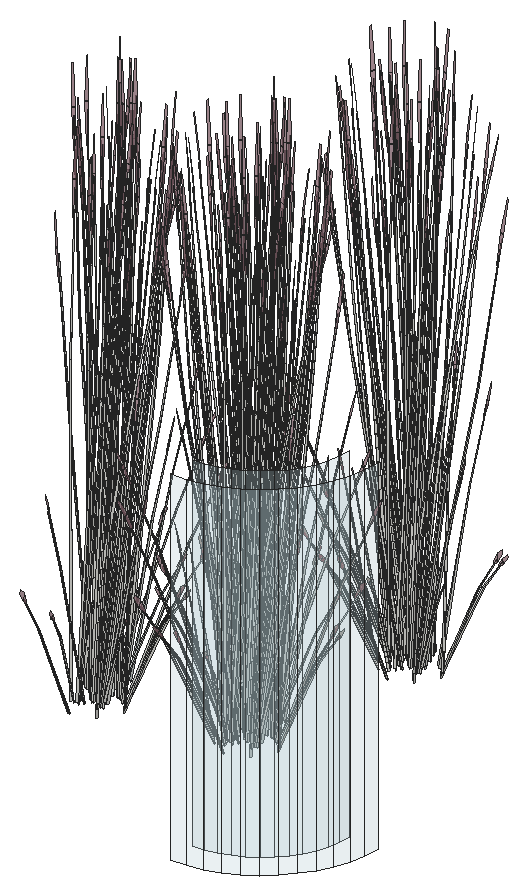
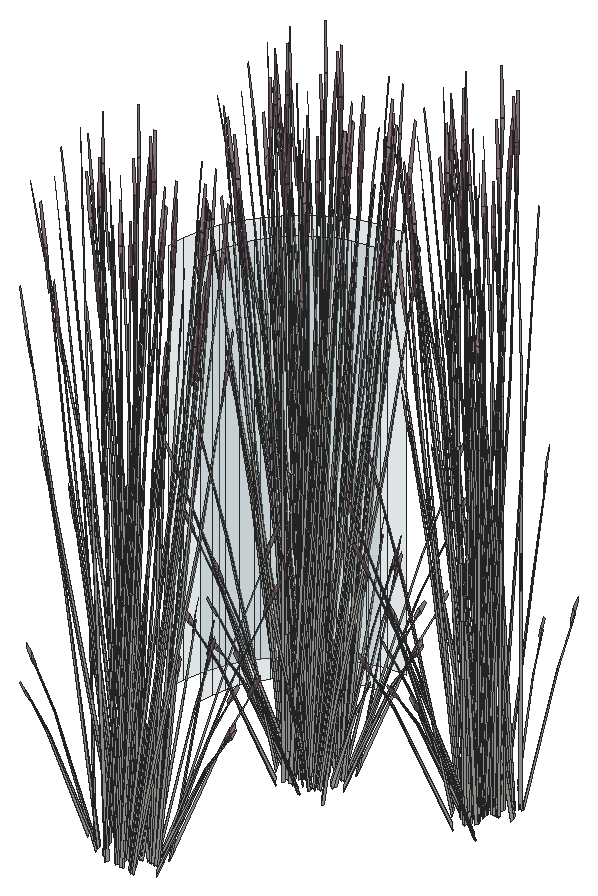
# SketchUp Ruby script. Lengths in inches.
U = 1.inch
M = Sketchup.active_model
def pt(a) = Geom::Point3d.new(a.map { |v| v * U })
def face(e, loops, mat)
  f = e.add_face(loops[0].map { |a| pt(a) })
  loops[1..].each { |l| e.add_face(l.map { |a| pt(a) }).erase! }
  f.material = f.back_material = mat if mat
  f
end
# faces: each face lists its corners as indices into pts; further lists are holes
def faces(e, pts, list, mat = nil) = list.each { |f| face(e, (f[0].is_a?(Array) ? f : [f]).map { |l| l.map { |i| pts[i] } }, mat) }
# xy, xz, yz: faces in a plane at the given z, y or x. An outline is a flat list of corners, or four numbers for a rectangle; further outlines are holes
def ring(l) = l.size == 4 ? [[l[0], l[1]], [l[2], l[1]], [l[2], l[3]], [l[0], l[3]]] : l.each_slice(2).to_a
def flat(e, list, mat, &to3) = list.each { |f| face(e, (f[0].is_a?(Array) ? f : [f]).map { |l| ring(l).map { |u, v| to3.(u, v) } }, mat) }
def xy(e, z, list, mat = nil) = flat(e, list, mat) { |x, y| [x, y, z] }
def xz(e, y, list, mat = nil) = flat(e, list, mat) { |x, z| [x, y, z] }
def yz(e, x, list, mat = nil) = flat(e, list, mat) { |y, z| [x, y, z] }
def lines(e, pts, list) = list.each { |a, b| e.add_line(pt(pts[a]), pt(pts[b])) }
# prism: a flat outline (further loops are holes) pulled along v
def prism(e, loops, v, mat = nil)
  f = face(e, loops, mat); d = Geom::Vector3d.new(v.map { |x| x * U })
  f.pushpull(f.normal.samedirection?(d) ? d.length : -d.length)
end
def box(e, o, s, mat = nil) = prism(e, [[o, [o[0] + s[0], o[1], o[2]], [o[0] + s[0], o[1] + s[1], o[2]], [o[0], o[1] + s[1], o[2]]]], [0, 0, s[2]], mat)
def at(x, y, z, deg = 0) = Geom::Transformation.translation(pt([x, y, z])) * Geom::Transformation.rotation(ORIGIN, Z_AXIS, deg.degrees)
def axes(o, x, y, z) = Geom::Transformation.new([*x, 0, *y, 0, *z, 0, *pt(o).to_a, 1])
def part(name) = M.definitions.add(name)
# library, detail: a bought-in or finely detailed component or shape, given as its bounding box
def library(name, o, s) = part(name).tap { |d| box(d.entities, o, s) }
def detail(e, o, s) = box(e.add_group.entities, o, s)
def put(e, d, t, mat = nil) = e.add_instance(d, t).tap { |i| i.material = mat if mat }
def group(e, t, mat = nil) = e.add_group.tap { |g| g.transformation = t; g.material = mat if mat }.entities
root = M.entities
M.materials.add("Glass_Safety_01").color = [204, 235, 244]
M.materials["Glass_Safety_01"].alpha = 0.25
M.materials.add("LightPink_Translucent").color = [144, 107, 117]
M.materials["LightPink_Translucent"].alpha = 0.75
c1 = part("blade")
p = [[2.15,0.21,22],[0,0.17,0],[0.09,0.45,0],[2.18,0.31,22],[2.29,0.31,22],[0.38,0.45,0],
  [2.48,0.24,33],[2.49,0.24,33],[2.48,0.22,33]]
faces(c1.entities,p,[[0,1,2,3],[4,5,2,3],[6,3,4,7],[8,0,3,6]])
c2 = part("seeds")
p = [[0.3,-0.1,1.38],[-0.01,-0.03,1.59],[-0.01,-0.03,0.03],[0.14,-0.07,-0.07],[0.29,-0.03,3],[0.15,0.01,3.11]]
faces(c2.entities,p,[[0,1,2,3],[1,0,4,5]],"LightPink_Translucent")
c3 = part("blade with seeds")
put(c3.entities,c1,at(0,0,0))
put(c3.entities,c2,axes([2.4,0.25,30.99],[1.5799,-0.05474,1.17369],[-0.12525,1.92788,0.29478],[-0.07173,-0.02425,1.56792]))
p = [[339,42,264],[340.56,42.125,264],[340.56,42.125,300],[339,42,300],[342.09,42.45,264],[342.09,42.45,300],
  [343.56,42.97,264],[343.56,42.97,300],[344.96,43.67,264],[344.96,43.67,300],[346.25,44.54,264],[346.25,44.54,300],
  [347.42,45.58,264],[347.42,45.58,300],[340.125,45.1,264],[338.95,45,264],[338.95,45,300],[340.125,45.1,300],
  [341.28,45.34,264],[341.28,45.34,300],[342.39,45.73,264],[342.39,45.73,300],[348.46,46.75,264],[348.46,46.75,300],
  [343.44,46.26,264],[343.44,46.26,300],[344.42,46.92,264],[344.42,46.92,300],[349.33,48.04,264],[349.33,48.04,300],
  [345.3,47.7,264],[345.3,47.7,300],[346.08,48.58,264],[346.08,48.58,300],[350.03,49.44,264],[350.03,49.44,300],
  [346.74,49.56,264],[346.74,49.56,300],[350.55,50.91,264],[350.55,50.91,300],[347.27,50.61,264],[347.27,50.61,300],
  [347.66,51.72,264],[347.66,51.72,300],[350.875,52.44,264],[350.875,52.44,300],[347.9,52.875,264],[347.9,52.875,300],
  [351,54,264],[351,54,300],[348,54.05,264],[348,54.05,300]]
faces(root,p,[[0,1,2,3],[1,4,5,2],[4,6,7,5],[6,8,9,7],[8,10,11,9],[10,12,13,11],[14,15,16,17],[18,14,17,19],
  [20,18,19,21],[12,22,23,13],[24,20,21,25],[26,24,25,27],[22,28,29,23],[30,26,27,31],[32,30,31,33],[28,34,35,29],
  [36,32,33,37],[34,38,39,35],[40,36,37,41],[42,40,41,43],[38,44,45,39],[46,42,43,47],[44,48,49,45],[50,46,47,51]],"Glass_Safety_01")
put(root,c3,axes([320.07,58.6,266.3],[0.14774,-0.54019,0.16428],[0.54062,0.15287,0.32672],[-0.09339,0.00263,1.49371]))
put(root,c3,axes([319.82,57.88,266.4375],[0.37783,0.32657,0.13483],[-0.31516,0.36844,-0.38503],[-0.08772,0.04981,1.18024]))
put(root,c3,axes([319.69,57.48,266.14],[-0.47569,-0.46784,-0.05709],[0.47598,-0.46812,0],[-0.01661,-0.01634,1.63492]))
put(root,c3,axes([319.8125,57.64,266.53],[0.55535,-0.03355,0.41661],[0.05022,0.55698,-0.2005],[-0.09942,0.05645,1.33761]))
put(root,c3,axes([319.95,58.92,266.17],[0.64025,0.17667,0.2864],[-0.16018,0.63149,-0.33981],[-0.10597,0.07904,1.53541]))
put(root,c3,axes([319.01,54.08,265.39],[-0.08578,0.01958,1.6421],[-0.47437,-0.22044,-0.25086],[0.00796,-0.18387,0.2797]))
put(root,c3,axes([320.22,58.89,266.31],[0.47863,-0.27177,0.46235],[0.28609,0.48733,0],[-0.10901,0.0619,1.46668]))
put(root,c3,axes([318.73,56.9375,266.2],[0.22235,0.6078,0.42607],[-0.63531,0.21135,0.16719],[0.00776,-0.11168,1.47927]))
put(root,c3,axes([318.625,56.86,266.06],[0.24813,-0.48978,-0.41661],[0.51557,0.23571,0.2005],[0,-0.1129,1.33761]))
put(root,c3,axes([319.26,58.44,266.05],[-0.16686,-0.46861,0],[0.47648,-0.16411,0],[0,0,1.4375]))
put(root,c3,axes([318.65,59.43,265.39],[0.08277,-0.02958,1.6421],[0.49786,0.16279,-0.25086],[0.01456,0.18348,0.2797]))
put(root,c3,axes([319.93,57.52,266.06],[-0.24813,0.48978,-0.41661],[-0.51557,-0.23571,0.2005],[0,0.1129,1.33761]))
put(root,c3,axes([320.91,57.22,266.3],[-0.40181,-0.39593,0.16428],[0.40492,-0.38402,0.32672],[-0.04438,0.08086,1.49371]))
put(root,c3,axes([319.53,56.99,266.05],[0,-0.62892,0],[0.63949,0,0],[0,0,1.6711]))
put(root,c3,axes([318.93,57.1,266.27],[0.57623,0.26344,0.22409],[-0.27732,0.5474,0.46562],[0,-0.12618,1.49497]))
put(root,c3,axes([319.85,57.24,266.13],[0,0.62861,-0.05249],[-0.63949,0,0],[0,0.01975,1.67027]))
put(root,c3,axes([318.74,56.74,266.53],[-0.55535,0.03355,0.41661],[-0.05022,-0.55698,-0.2005],[0.09942,-0.05645,1.33761]))
put(root,c3,axes([318.49,55.78,266.3],[-0.14774,0.54019,0.16428],[-0.54062,-0.15287,0.32672],[0.09339,-0.00263,1.49371]))
put(root,c3,axes([319.54,58.46,266.13],[0.22235,0.62444,-0.05599],[-0.63531,0.21881,0],[0.00776,0.02181,1.60327]))
put(root,c3,axes([318.22,55.11,266.21],[-0.31974,-0.54466,0],[0.53494,-0.30375,-0.48057],[0.12184,-0.06918,1.52448]))
put(root,c3,axes([321.38,57.64,266.05],[-0.63917,-0.00435,-0.04634],[0,-0.60749,0.46507],[-0.02009,0.13829,1.47457]))
put(root,c3,axes([320.12,55.8125,266.3],[-0.54955,0.14427,0.16428],[-0.1357,-0.53689,0.32672],[0.04901,0.07823,1.49371]))
put(root,c3,axes([319.56,53.8,266.58],[0.06561,0.31695,1.06958],[-0.36394,-0.17555,0.78586],[0.03916,-0.16229,0.23558]))
put(root,c3,axes([319.22,56.59,266.2],[-0.42403,0.49328,0.42607],[-0.50377,-0.43543,0.16719],[0.10223,-0.04923,1.47927]))
put(root,c3,axes([319.95,57.37,266.0625],[0.35699,0.35109,0],[-0.35699,0.35109,0],[0,0,1.57621]))
put(root,c3,axes([319.94,56.96,266.53],[0.24813,-0.48978,0.41661],[0.51557,0.23571,-0.2005],[0,0.1129,1.33761]))
put(root,c3,axes([319.73,58.66,266.05],[0.51557,0.24403,0],[-0.24813,0.50705,0],[0,0,1.62917]))
put(root,c3,axes([319.77,56.84,266.22],[-0.64638,-0.11452,0.45814],[0.13155,-0.64678,0.17978],[0.09446,0.06245,1.59061]))
put(root,c3,axes([321.24,57.73,265.89],[-0.35699,0.33913,-0.28847],[-0.35699,-0.33913,0.28847],[0,0.10923,1.29413]))
put(root,c3,axes([320.22,57.66,265.95],[0.18752,0.49766,-0.6445],[-0.54017,0.17923,-0.16915],[0.02073,0.16852,1.42262]))
put(root,c3,axes([319.96,57.13,266.05],[0.57217,0,0],[0,0.56272,0],[0,0,1.66132]))
put(root,c3,axes([319.41,56.51,266.53],[-0.30722,-0.45622,0.41661],[0.46535,-0.32126,-0.2005],[0.09942,0.05645,1.33761]))
put(root,c3,axes([318.85,56.62,266.48],[-0.05959,-0.62022,-0.27094],[0.62068,-0.0375,-0.46562],[0.1093,-0.08261,1.4872]))
put(root,c3,axes([320.16,57.07,266.4375],[0.47648,-0.15851,0.13483],[0.16686,0.45265,-0.38503],[0,0.09962,1.18024]))
put(root,c3,axes([319.99,57.11,266.48],[0.57594,0.25935,-0.27094],[-0.27732,0.5474,-0.46562],[0.0181,0.1344,1.4872]))
put(root,c3,axes([318.77,55.25,265.89],[0.47712,0.13449,-0.28847],[-0.12013,0.47362,0.28847],[0.09619,-0.05462,1.29413]))
put(root,c3,axes([320.1,54.67,266.41],[-0.14537,0.11002,1.33163],[-0.43536,-0.19256,-0.28638],[0.0807,-0.23948,0.56934]))
put(root,c3,axes([321.24,57.23,266.31],[0,-0.54355,0.46235],[0.57217,0,0],[0,0.1238,1.46668]))
put(root,c3,axes([321.49,57.74,265.88],[0,0.54355,-0.46235],[-0.57217,0,0],[0,0.1238,1.46668]))
put(root,c3,axes([318.66,55.03,265.88],[0.47863,-0.27177,-0.46235],[0.28609,0.48733,0],[0.10901,-0.0619,1.46668]))
put(root,c3,axes([319.62,56.38,266.4375],[0.09866,-0.48509,0.13483],[0.48202,0.0842,-0.38503],[0.08772,0.04981,1.18024]))
put(root,c3,axes([320.3,55.54,266.31],[-0.47863,-0.27177,0.46235],[0.28609,-0.48733,0],[0.10901,0.0619,1.46668]))
put(root,c3,axes([319.88,58.375,266.03],[0.53691,-0.18442,-0.17877],[0.18866,0.53125,0.00007],[0.05927,-0.02038,1.61933]))
put(root,c3,axes([319.89,56.8,266.06],[0.30722,0.45622,-0.41661],[-0.46535,0.32126,0.2005],[0.09942,0.05645,1.33761]))
put(root,c3,axes([320.76,58.87,266.58],[-0.28795,-0.15629,1.06958],[0.37181,-0.1588,0.78586],[0.10029,0.13452,0.23558]))
put(root,c3,axes([319.74,58.7,266.41],[0.00902,-0.18018,1.33163],[0.43127,-0.20126,-0.28638],[0.13313,0.21566,0.56934]))
put(root,c3,axes([319.22,56.15,265.92],[0.34446,-0.40855,-0.58063],[0.42791,0.37046,-0.15239],[0.13803,-0.10191,1.28164]))
put(root,c3,axes([320.73,55.78,265.89],[0.12013,0.47362,-0.28847],[-0.47712,0.13449,0.28847],[0.09619,0.05462,1.29413]))
put(root,c3,axes([321.63,57.33,266.21],[0.63949,0,0],[0,0.60749,-0.48057],[0,0.13836,1.52448]))
put(root,c3,axes([319.57,56.54,266.48],[0.51635,-0.36087,-0.27094],[0.34336,0.5099,-0.46562],[0.1274,0.05178,1.4872]))
put(root,c3,axes([320.81,59.58,266.48],[-0.32795,-0.01705,0.97832],[0.21658,-0.36206,0.54015],[0.12956,0.12863,0.76741]))
put(root,c3,axes([318.26,56.22,265.48],[-0.50338,0.21762,1.20058],[-0.16022,-0.62439,0.4665],[0.30911,0.01039,1.36553]))
put(root,c3,axes([320.58,55.25,266.21],[0.31974,-0.54466,0],[0.53494,0.30375,-0.48057],[0.12184,0.06918,1.52448]))
put(root,c3,axes([321.11,55.01,265.39],[-0.07655,-0.04282,1.6421],[-0.19662,-0.47839,-0.25086],[0.13264,-0.12982,0.2797]))
put(root,c3,axes([320.87,55.58,265.88],[0.47863,0.27177,-0.46235],[-0.28609,0.48733,0],[0.10901,0.0619,1.46668]))
put(root,c3,axes([320.84,59.45,265.39],[0.03726,-0.07847,1.6421],[0.46909,-0.23111,-0.25086],[0.14221,0.11962,0.2797]))
put(root,c3,axes([320.17,56.62,265.92],[0.53199,0.08911,-0.58063],[-0.11226,0.54969,-0.15239],[0.15876,0.06661,1.28164]))
put(root,c3,axes([322.43,56.94,266.11],[-0.31706,-0.34757,-0.06041],[0.34725,-0.31847,-0.27392],[0.09839,-0.02242,0.90349]))
put(root,c3,axes([321.71,55.18,266.58],[-0.17034,0.27669,1.06958],[-0.14642,-0.37174,0.78586],[0.14069,-0.09315,0.23558]))
put(root,c3,axes([322.52,57.58,266.58],[-0.31598,0.08973,1.06958],[0.14873,-0.37085,0.78586],[0.16763,0.02538,0.23558]))
put(root,c3,axes([321.5,55.97,266.41],[-0.1827,-0.0161,1.33163],[-0.18717,-0.43188,-0.28638],[0.22444,-0.12218,0.56934]))
put(root,c3,axes([321.83,57.4,265.85],[-0.32938,0.06523,1.31842],[-0.05243,-0.51922,0.07547],[0.2307,-0.07859,0.75023]))
put(root,c3,axes([322.19,57.06,265.39],[-0.02673,-0.08252,1.6421],[0.18538,-0.48271,-0.25086],[0.187,-0.00694,0.2797]))
put(root,c3,axes([330.18,60.87,266.41],[0.17773,0.04462,1.33163],[0.11455,0.45576,-0.28638],[-0.24142,0.08531,0.56934]))
put(root,c3,axes([321.93,58.18,266.41],[-0.12317,-0.13368,1.33163],[0.16025,-0.44223,-0.28638],[0.24919,0.05991,0.56934]))
put(root,c3,axes([330.86,58.66,266.41],[0.09985,0.15133,1.33163],[-0.23008,0.41134,-0.28638],[-0.23625,-0.09832,0.56934]))
put(root,c3,axes([330.51,59.68,265.39],[0.01297,0.08566,1.6421],[-0.26146,0.44735,-0.25086],[-0.18572,-0.02255,0.2797]))
put(root,c3,axes([329.81,61.82,266.58],[0.21313,-0.24635,1.06958],[0.0841,0.38999,0.78586],[-0.15402,0.06983,0.23558]))
put(root,c3,axes([330.37,62.08,265.39],[0.0686,0.0543,1.6421],[0.11632,0.50315,-0.25086],[-0.15204,0.10729,0.2797]))
put(root,c3,axes([330.27,59.12,266.58],[0.3265,-0.03889,1.06958],[-0.20711,0.3427,0.78586],[-0.16135,-0.05141,0.23558]))
put(root,c3,axes([332.22,60.45,265.92],[-0.53199,-0.08911,-0.58063],[0.11226,-0.54969,-0.15239],[-0.15876,-0.06661,1.28164]))
put(root,c3,axes([331.52,61.49,265.88],[-0.47863,-0.27177,-0.46235],[0.28609,-0.48733,0],[-0.10901,-0.0619,1.46668]))
put(root,c3,axes([331.31,57.45,265.39],[-0.04954,0.0716,1.6421],[-0.50062,0.15438,-0.25086],[-0.12094,-0.14044,0.2797]))
put(root,c3,axes([331.8125,61.82,266.21],[-0.31974,0.54466,0],[-0.53494,-0.30375,-0.48057],[-0.12184,-0.06918,1.52448]))
put(root,c3,axes([333.5625,76.51,266.41],[0.09985,0.15133,1.33163],[-0.23008,0.41134,-0.28638],[-0.23625,-0.09832,0.56934]))
put(root,c3,axes([331.23,62.61,266.41],[0.16138,-0.08575,1.33163],[0.39845,0.25854,-0.28638],[-0.1186,0.22371,0.56934]))
put(root,c3,axes([331,57.72,265.98],[-0.14753,0.44383,-0.03625],[-0.45406,-0.13653,-0.16435],[-0.06894,-0.07259,0.54209]))
put(root,c3,axes([331.68,57.16,266.41],[-0.03097,0.17781,1.33163],[-0.45273,0.14885,-0.28638],[-0.10583,-0.22982,0.56934]))
put(root,c3,axes([332.82,60.54,266.48],[-0.51635,0.36087,-0.27094],[-0.34336,-0.5099,-0.46562],[-0.1274,-0.05178,1.4872]))
put(root,c3,axes([333.2,77.53,265.39],[0.01297,0.08566,1.6421],[-0.26146,0.44735,-0.25086],[-0.18572,-0.02255,0.2797]))
put(root,c3,axes([330.76,59.75,266.21],[-0.63949,0,0],[0,-0.60749,-0.48057],[0,-0.13836,1.52448]))
put(root,c3,axes([331.65,61.29,265.89],[-0.12013,-0.47362,-0.28847],[0.47712,-0.13449,0.28847],[-0.09619,-0.05462,1.29413]))
put(root,c3,axes([333.16,60.93,265.92],[-0.34446,0.40855,-0.58063],[-0.42791,-0.37046,-0.15239],[-0.13803,0.10191,1.28164]))
put(root,c3,axes([331.25,59.59,266.17],[-0.47569,0.45698,0.2864],[-0.47598,-0.45217,-0.33981],[-0.01661,-0.12977,1.53541]))
put(root,c3,axes([331.52,56.875,266.58],[0.26677,0.18918,1.06958],[-0.38851,0.11372,0.78586],[-0.08313,-0.14539,0.23558]))
put(root,c3,axes([333.4,60.7,266.3],[-0.49938,-0.43748,-0.23459],[0.42021,-0.49126,0.51337],[-0.13447,0.05118,1.56642]))
put(root,c3,axes([332.49,60.28,266.06],[-0.30722,-0.45622,-0.41661],[0.46535,-0.32126,0.2005],[-0.09942,-0.05645,1.33761]))
put(root,c3,axes([332.97,76.97,266.58],[0.3265,-0.03889,1.06958],[-0.20711,0.3427,0.78586],[-0.16135,-0.05141,0.23558]))
put(root,c3,axes([331.61,62.9,266.58],[-0.01324,-0.32319,1.06958],[0.33072,0.23052,0.78586],[-0.06504,0.15405,0.23558]))
put(root,c3,axes([333.15,60.61,266.06],[-0.55535,0.03355,-0.41661],[-0.05022,-0.55698,0.2005],[-0.09942,0.05645,1.33761]))
put(root,c3,axes([332.09,61.54,266.31],[0.47863,0.27177,0.46235],[-0.28609,0.48733,0],[-0.10901,-0.0619,1.46668]))
put(root,c3,axes([332.54,60.54,266.27],[0.13555,-0.64407,-0.21817],[0.64269,0.11227,0.47743],[-0.1123,-0.08895,1.45677]))
put(root,c3,axes([332.77,60.69,266.4375],[-0.09866,0.48509,0.13483],[-0.48202,-0.0842,-0.38503],[-0.08772,-0.04981,1.18024]))
put(root,c3,axes([333.73,62.04,265.88],[-0.47863,0.27177,-0.46235],[-0.28609,-0.48733,0],[-0.10901,0.0619,1.46668]))
put(root,c3,axes([330.9,59.34,265.88],[0,-0.54355,-0.46235],[0.57217,0,0],[0,-0.1238,1.46668]))
put(root,c3,axes([331.14,59.84,266.31],[0,0.54355,0.46235],[-0.57217,0,0],[0,-0.1238,1.46668]))
put(root,c3,axes([333.76,61.9,266.04],[-0.31576,-0.54657,-0.04789],[0.53494,-0.30375,0.48057],[-0.13182,0.05204,1.52373]))
put(root,c3,axes([333.62,61.83,265.89],[-0.47712,-0.13449,-0.28847],[0.12013,-0.47362,0.28847],[-0.09619,0.05462,1.29413]))
put(root,c3,axes([332.39,59.97,266.48],[-0.57594,-0.25935,-0.27094],[0.27732,-0.5474,-0.46562],[-0.0181,-0.1344,1.4872]))
put(root,c3,axes([334.92,78.3,265.92],[-0.53199,-0.08911,-0.58063],[0.11226,-0.54969,-0.15239],[-0.15876,-0.06661,1.28164]))
put(root,c3,axes([331.34,62.2,266.63],[0.46459,-0.09625,0.0606],[0.10681,0.38778,-0.80367],[-0.02945,0.1963,0.72038]))
put(root,c3,axes([333.54,60.46,266.48],[0.05959,0.62022,-0.27094],[-0.62068,0.0375,-0.46562],[-0.1093,0.08261,1.4872]))
put(root,c3,axes([332.14,59.41,265.95],[-0.21003,-0.55738,-0.65031],[0.60499,-0.20074,-0.17068],[-0.02321,-0.18874,1.43544]))
put(root,c3,axes([334.22,79.34,265.88],[-0.47863,-0.27177,-0.46235],[0.28609,-0.48733,0],[-0.10901,-0.0619,1.46668]))
put(root,c3,axes([334.01,75.3,265.39],[-0.04954,0.0716,1.6421],[-0.50062,0.15438,-0.25086],[-0.12094,-0.14044,0.2797]))
put(root,c3,axes([331.14,59.35,265.89],[0.35699,-0.33913,-0.28847],[0.35699,0.33913,0.28847],[0,-0.10923,1.29413]))
put(root,c3,axes([332.76,57.16,265.98],[-0.35341,0.31182,-0.03625],[-0.32382,-0.34152,-0.16435],[-0.0228,-0.09677,0.54209]))
put(root,c3,axes([332.61,60.23,266.2],[0.64638,0.11452,0.42607],[-0.13155,0.64678,0.16719],[-0.09446,-0.06245,1.47927]))
put(root,c3,axes([332.45,60.11,266.53],[-0.24813,0.48978,0.41661],[-0.51557,-0.23571,-0.2005],[0,-0.1129,1.33761]))
put(root,c3,axes([333.7,75.57,265.98],[-0.14753,0.44383,-0.03625],[-0.45406,-0.13653,-0.16435],[-0.06894,-0.07259,0.54209]))
put(root,c3,axes([332.27,61.26,266.3],[0.54955,-0.14427,0.16428],[0.1357,0.53689,0.32672],[-0.04901,-0.07823,1.49371]))
put(root,c3,axes([332.97,61.35,266.05],[-0.51557,-0.24403,0],[0.24813,-0.50705,0],[0,0,1.51513]))
put(root,c3,axes([334.17,61.96,266.21],[0.31974,0.54466,0],[-0.53494,0.30375,-0.48057],[-0.12184,0.06918,1.52448]))
put(root,c3,axes([334.375,75.01,266.41],[-0.03097,0.17781,1.33163],[-0.45273,0.14885,-0.28638],[-0.10583,-0.22982,0.56934]))
put(root,c3,axes([335.52,78.38,266.48],[-0.51635,0.36087,-0.27094],[-0.34336,-0.5099,-0.46562],[-0.1274,-0.05178,1.4872]))
put(root,c3,axes([333.45,77.6,266.21],[-0.63949,0,0],[0,-0.60749,-0.48057],[0,-0.13836,1.52448]))
put(root,c3,axes([334.35,79.14,265.89],[-0.12013,-0.47362,-0.28847],[0.47712,-0.13449,0.28847],[-0.09619,-0.05462,1.29413]))
put(root,c3,axes([333.9,61.29,266.3],[0.14774,-0.54019,0.16428],[0.54062,0.15287,0.32672],[-0.09339,0.00263,1.49371]))
put(root,c3,axes([333.65,60.58,266.4375],[0.37783,0.32657,0.13483],[-0.31516,0.36844,-0.38503],[-0.08772,0.04981,1.18024]))
put(root,c3,axes([333.52,60.17,266.14],[-0.47569,-0.46784,-0.05709],[0.47598,-0.46812,0],[-0.01661,-0.01634,1.63492]))
put(root,c3,axes([333.64,60.34,266.53],[0.55535,-0.03355,0.41661],[0.05022,0.55698,-0.2005],[-0.09942,0.05645,1.33761]))
put(root,c3,axes([333.78,61.62,266.17],[0.64025,0.17667,0.2864],[-0.16018,0.63149,-0.33981],[-0.10597,0.07904,1.53541]))
put(root,c3,axes([332.84,56.77,265.39],[-0.08578,0.01958,1.6421],[-0.47437,-0.22044,-0.25086],[0.00796,-0.18387,0.2797]))
put(root,c3,axes([334.05,61.58,266.31],[0.47863,-0.27177,0.46235],[0.28609,0.48733,0],[-0.10901,0.0619,1.46668]))
put(root,c3,axes([333.95,77.4375,266.17],[-0.47569,0.45698,0.2864],[-0.47598,-0.45217,-0.33981],[-0.01661,-0.12977,1.53541]))
put(root,c3,axes([332.56,59.64,266.2],[0.22235,0.6078,0.42607],[-0.63531,0.21135,0.16719],[0.00776,-0.11168,1.47927]))
put(root,c3,axes([332.46,59.56,266.06],[0.24813,-0.48978,-0.41661],[0.51557,0.23571,0.2005],[0,-0.1129,1.33761]))
put(root,c3,axes([333.09,61.14,266.05],[-0.16686,-0.46861,0],[0.47648,-0.16411,0],[0,0,1.4375]))
put(root,c3,axes([332.49,62.125,265.39],[0.08277,-0.02958,1.6421],[0.49786,0.16279,-0.25086],[0.01456,0.18348,0.2797]))
put(root,c3,axes([334.22,74.73,266.58],[0.26677,0.18918,1.06958],[-0.38851,0.11372,0.78586],[-0.08313,-0.14539,0.23558]))
put(root,c3,axes([336.1,78.55,266.3],[-0.49938,-0.43748,-0.23459],[0.42021,-0.49126,0.51337],[-0.13447,0.05118,1.56642]))
put(root,c3,axes([335.19,78.13,266.06],[-0.30722,-0.45622,-0.41661],[0.46535,-0.32126,0.2005],[-0.09942,-0.05645,1.33761]))
put(root,c3,axes([333.76,60.21,266.06],[-0.24813,0.48978,-0.41661],[-0.51557,-0.23571,0.2005],[0,0.1129,1.33761]))
put(root,c3,axes([334.78,79.39,266.31],[0.47863,0.27177,0.46235],[-0.28609,0.48733,0],[-0.10901,-0.0619,1.46668]))
put(root,c3,axes([334.75,59.92,266.3],[-0.40181,-0.39593,0.16428],[0.40492,-0.38402,0.32672],[-0.04438,0.08086,1.49371]))
put(root,c3,axes([333.36,59.6875,266.05],[0,-0.62892,0],[0.63949,0,0],[0,0,1.6711]))
put(root,c3,axes([335.24,78.39,266.27],[0.13555,-0.64407,-0.21817],[0.64269,0.11227,0.47743],[-0.1123,-0.08895,1.45677]))
put(root,c3,axes([332.76,59.8,266.27],[0.57623,0.26344,0.22409],[-0.27732,0.5474,0.46562],[0,-0.12618,1.49497]))
put(root,c3,axes([333.68,59.9375,266.13],[0,0.62861,-0.05249],[-0.63949,0,0],[0,0.01975,1.67027]))
put(root,c3,axes([332.58,59.43,266.53],[-0.55535,0.03355,0.41661],[-0.05022,-0.55698,-0.2005],[0.09942,-0.05645,1.33761]))
put(root,c3,axes([335.47,78.54,266.4375],[-0.09866,0.48509,0.13483],[-0.48202,-0.0842,-0.38503],[-0.08772,-0.04981,1.18024]))
put(root,c3,axes([332.32,58.48,266.3],[-0.14774,0.54019,0.16428],[-0.54062,-0.15287,0.32672],[0.09339,-0.00263,1.49371]))
put(root,c3,axes([333.375,61.15,266.13],[0.22235,0.62444,-0.05599],[-0.63531,0.21881,0],[0.00776,0.02181,1.60327]))
put(root,c3,axes([333.6,77.19,265.88],[0,-0.54355,-0.46235],[0.57217,0,0],[0,-0.1238,1.46668]))
put(root,c3,axes([333.84,77.69,266.31],[0,0.54355,0.46235],[-0.57217,0,0],[0,-0.1238,1.46668]))
put(root,c3,axes([332.05,57.8125,266.21],[-0.31974,-0.54466,0],[0.53494,-0.30375,-0.48057],[0.12184,-0.06918,1.52448]))
put(root,c3,axes([335.21,60.33,266.05],[-0.63917,-0.00435,-0.04634],[0,-0.60749,0.46507],[-0.02009,0.13829,1.47457]))
put(root,c3,axes([335.09,77.8125,266.48],[-0.57594,-0.25935,-0.27094],[0.27732,-0.5474,-0.46562],[-0.0181,-0.1344,1.4872]))
put(root,c3,axes([333.95,58.51,266.3],[-0.54955,0.14427,0.16428],[-0.1357,-0.53689,0.32672],[0.04901,0.07823,1.49371]))
put(root,c3,axes([333.39,56.5,266.58],[0.06561,0.31695,1.06958],[-0.36394,-0.17555,0.78586],[0.03916,-0.16229,0.23558]))
put(root,c3,axes([333.05,59.29,266.2],[-0.42403,0.49328,0.42607],[-0.50377,-0.43543,0.16719],[0.10223,-0.04923,1.47927]))
put(root,c3,axes([333.78,60.07,266.0625],[0.35699,0.35109,0],[-0.35699,0.35109,0],[0,0,1.57621]))
put(root,c3,axes([334.83,77.26,265.95],[-0.21003,-0.55738,-0.65031],[0.60499,-0.20074,-0.17068],[-0.02321,-0.18874,1.43544]))
put(root,c3,axes([333.77,59.66,266.53],[0.24813,-0.48978,0.41661],[0.51557,0.23571,-0.2005],[0,0.1129,1.33761]))
put(root,c3,axes([333.56,61.36,266.05],[0.51557,0.24403,0],[-0.24813,0.50705,0],[0,0,1.62917]))
put(root,c3,axes([333.61,59.54,266.22],[-0.64638,-0.11452,0.45814],[0.13155,-0.64678,0.17978],[0.09446,0.06245,1.59061]))
put(root,c3,axes([333.84,77.2,265.89],[0.35699,-0.33913,-0.28847],[0.35699,0.33913,0.28847],[0,-0.10923,1.29413]))
put(root,c3,axes([335.45,75,265.98],[-0.35341,0.31182,-0.03625],[-0.32382,-0.34152,-0.16435],[-0.0228,-0.09677,0.54209]))
put(root,c3,axes([335.08,60.42,265.89],[-0.35699,0.33913,-0.28847],[-0.35699,-0.33913,0.28847],[0,0.10923,1.29413]))
put(root,c3,axes([335.31,78.08,266.2],[0.64638,0.11452,0.42607],[-0.13155,0.64678,0.16719],[-0.09446,-0.06245,1.47927]))
put(root,c3,axes([334.06,60.36,265.95],[0.18752,0.49766,-0.6445],[-0.54017,0.17923,-0.16915],[0.02073,0.16852,1.42262]))
put(root,c3,axes([333.79,59.83,266.05],[0.57217,0,0],[0,0.56272,0],[0,0,1.66132]))
put(root,c3,axes([335.14,77.96,266.53],[-0.24813,0.48978,0.41661],[-0.51557,-0.23571,-0.2005],[0,-0.1129,1.33761]))
put(root,c3,axes([333.24,59.21,266.53],[-0.30722,-0.45622,0.41661],[0.46535,-0.32126,-0.2005],[0.09942,0.05645,1.33761]))
put(root,c3,axes([332.68,59.32,266.48],[-0.05959,-0.62022,-0.27094],[0.62068,-0.0375,-0.46562],[0.1093,-0.08261,1.4872]))
put(root,c3,axes([333.99,59.77,266.4375],[0.47648,-0.15851,0.13483],[0.16686,0.45265,-0.38503],[0,0.09962,1.18024]))
put(root,c3,axes([334.96,79.11,266.3],[0.54955,-0.14427,0.16428],[0.1357,0.53689,0.32672],[-0.04901,-0.07823,1.49371]))
put(root,c3,axes([333.83,59.81,266.48],[0.57594,0.25935,-0.27094],[-0.27732,0.5474,-0.46562],[0.0181,0.1344,1.4872]))
put(root,c3,axes([335.67,79.2,266.05],[-0.51557,-0.24403,0],[0.24813,-0.50705,0],[0,0,1.51513]))
put(root,c3,axes([332.6,57.94,265.89],[0.47712,0.13449,-0.28847],[-0.12013,0.47362,0.28847],[0.09619,-0.05462,1.29413]))
put(root,c3,axes([333.93,57.37,266.41],[-0.14537,0.11002,1.33163],[-0.43536,-0.19256,-0.28638],[0.0807,-0.23948,0.56934]))
put(root,c3,axes([335.08,59.93,266.31],[0,-0.54355,0.46235],[0.57217,0,0],[0,0.1238,1.46668]))
put(root,c3,axes([335.32,60.44,265.88],[0,0.54355,-0.46235],[-0.57217,0,0],[0,0.1238,1.46668]))
put(root,c3,axes([332.49,57.73,265.88],[0.47863,-0.27177,-0.46235],[0.28609,0.48733,0],[0.10901,-0.0619,1.46668]))
put(root,c3,axes([336.6,79.14,266.3],[0.14774,-0.54019,0.16428],[0.54062,0.15287,0.32672],[-0.09339,0.00263,1.49371]))
put(root,c3,axes([333.45,59.08,266.4375],[0.09866,-0.48509,0.13483],[0.48202,0.0842,-0.38503],[0.08772,0.04981,1.18024]))
put(root,c3,axes([336.21,78.02,266.14],[-0.47569,-0.46784,-0.05709],[0.47598,-0.46812,0],[-0.01661,-0.01634,1.63492]))
put(root,c3,axes([335.54,74.62,265.39],[-0.08578,0.01958,1.6421],[-0.47437,-0.22044,-0.25086],[0.00796,-0.18387,0.2797]))
put(root,c3,axes([334.13,58.23,266.31],[-0.47863,-0.27177,0.46235],[0.28609,-0.48733,0],[0.10901,0.0619,1.46668]))
put(root,c3,axes([335.25,77.48,266.2],[0.22235,0.6078,0.42607],[-0.63531,0.21135,0.16719],[0.00776,-0.11168,1.47927]))
put(root,c3,axes([333.72,61.07,266.03],[0.53691,-0.18442,-0.17877],[0.18866,0.53125,0.00007],[0.05927,-0.02038,1.61933]))
put(root,c3,axes([335.15,77.41,266.06],[0.24813,-0.48978,-0.41661],[0.51557,0.23571,0.2005],[0,-0.1129,1.33761]))
put(root,c3,axes([335.79,78.99,266.05],[-0.16686,-0.46861,0],[0.47648,-0.16411,0],[0,0,1.4375]))
put(root,c3,axes([333.73,59.49,266.06],[0.30722,0.45622,-0.41661],[-0.46535,0.32126,0.2005],[0.09942,0.05645,1.33761]))
put(root,c3,axes([334.6,61.5625,266.58],[-0.28795,-0.15629,1.06958],[0.37181,-0.1588,0.78586],[0.10029,0.13452,0.23558]))
put(root,c3,axes([333.57,61.4,266.41],[0.00902,-0.18018,1.33163],[0.43127,-0.20126,-0.28638],[0.13313,0.21566,0.56934]))
put(root,c3,axes([333.06,58.84,265.92],[0.34446,-0.40855,-0.58063],[0.42791,0.37046,-0.15239],[0.13803,-0.10191,1.28164]))
put(root,c3,axes([337.44,77.76,266.3],[-0.40181,-0.39593,0.16428],[0.40492,-0.38402,0.32672],[-0.04438,0.08086,1.49371]))
put(root,c3,axes([336.05,77.54,266.05],[0,-0.62892,0],[0.63949,0,0],[0,0,1.6711]))
put(root,c3,axes([335.46,77.65,266.27],[0.57623,0.26344,0.22409],[-0.27732,0.5474,0.46562],[0,-0.12618,1.49497]))
put(root,c3,axes([335.27,77.28,266.53],[-0.55535,0.03355,0.41661],[-0.05022,-0.55698,-0.2005],[0.09942,-0.05645,1.33761]))
put(root,c3,axes([335.02,76.33,266.3],[-0.14774,0.54019,0.16428],[-0.54062,-0.15287,0.32672],[0.09339,-0.00263,1.49371]))
put(root,c3,axes([334.57,58.48,265.89],[0.12013,0.47362,-0.28847],[-0.47712,0.13449,0.28847],[0.09619,0.05462,1.29413]))
put(root,c3,axes([335.46,60.02,266.21],[0.63949,0,0],[0,0.60749,-0.48057],[0,0.13836,1.52448]))
put(root,c3,axes([333.4,59.24,266.48],[0.51635,-0.36087,-0.27094],[0.34336,0.5099,-0.46562],[0.1274,0.05178,1.4872]))
put(root,c3,axes([334.64,62.27,266.48],[-0.32795,-0.01705,0.97832],[0.21658,-0.36206,0.54015],[0.12956,0.12863,0.76741]))
put(root,c3,axes([334.75,75.66,266.21],[-0.31974,-0.54466,0],[0.53494,-0.30375,-0.48057],[0.12184,-0.06918,1.52448]))
put(root,c3,axes([336.65,76.36,266.3],[-0.54955,0.14427,0.16428],[-0.1357,-0.53689,0.32672],[0.04901,0.07823,1.49371]))
put(root,c3,axes([336.09,74.34,266.58],[0.06561,0.31695,1.06958],[-0.36394,-0.17555,0.78586],[0.03916,-0.16229,0.23558]))
put(root,c3,axes([335.75,77.14,266.2],[-0.42403,0.49328,0.42607],[-0.50377,-0.43543,0.16719],[0.10223,-0.04923,1.47927]))
put(root,c3,axes([336.48,77.92,266.0625],[0.35699,0.35109,0],[-0.35699,0.35109,0],[0,0,1.57621]))
put(root,c3,axes([332.09,58.91,265.48],[-0.50338,0.21762,1.20058],[-0.16022,-0.62439,0.4665],[0.30911,0.01039,1.36553]))
put(root,c3,axes([336.3,77.39,266.22],[-0.64638,-0.11452,0.45814],[0.13155,-0.64678,0.17978],[0.09446,0.06245,1.59061]))
put(root,c3,axes([334.41,57.95,266.21],[0.31974,-0.54466,0],[0.53494,0.30375,-0.48057],[0.12184,0.06918,1.52448]))
put(root,c3,axes([334.94,57.71,265.39],[-0.07655,-0.04282,1.6421],[-0.19662,-0.47839,-0.25086],[0.13264,-0.12982,0.2797]))
put(root,c3,axes([334.7,58.28,265.88],[0.47863,0.27177,-0.46235],[-0.28609,0.48733,0],[0.10901,0.0619,1.46668]))
put(root,c3,axes([336.49,77.68,266.05],[0.57217,0,0],[0,0.56272,0],[0,0,1.66132]))
put(root,c3,axes([335.9375,77.06,266.53],[-0.30722,-0.45622,0.41661],[0.46535,-0.32126,-0.2005],[0.09942,0.05645,1.33761]))
put(root,c3,axes([335.38,77.16,266.48],[-0.05959,-0.62022,-0.27094],[0.62068,-0.0375,-0.46562],[0.1093,-0.08261,1.4872]))
put(root,c3,axes([334.68,62.14,265.39],[0.03726,-0.07847,1.6421],[0.46909,-0.23111,-0.25086],[0.14221,0.11962,0.2797]))
put(root,c3,axes([334,59.32,265.92],[0.53199,0.08911,-0.58063],[-0.11226,0.54969,-0.15239],[0.15876,0.06661,1.28164]))
put(root,c3,axes([336.27,59.64,266.11],[-0.31706,-0.34757,-0.06041],[0.34725,-0.31847,-0.27392],[0.09839,-0.02242,0.90349]))
put(root,c3,axes([335.3,75.79,265.89],[0.47712,0.13449,-0.28847],[-0.12013,0.47362,0.28847],[0.09619,-0.05462,1.29413]))
put(root,c3,axes([336.625,75.22,266.41],[-0.14537,0.11002,1.33163],[-0.43536,-0.19256,-0.28638],[0.0807,-0.23948,0.56934]))
put(root,c3,axes([335.54,57.87,266.58],[-0.17034,0.27669,1.06958],[-0.14642,-0.37174,0.78586],[0.14069,-0.09315,0.23558]))
put(root,c3,axes([335.18,75.58,265.88],[0.47863,-0.27177,-0.46235],[0.28609,0.48733,0],[0.10901,-0.0619,1.46668]))
put(root,c3,axes([336.14,76.93,266.4375],[0.09866,-0.48509,0.13483],[0.48202,0.0842,-0.38503],[0.08772,0.04981,1.18024]))
put(root,c3,axes([336.83,76.08,266.31],[-0.47863,-0.27177,0.46235],[0.28609,-0.48733,0],[0.10901,0.0619,1.46668]))
put(root,c3,axes([336.41,78.92,266.03],[0.53691,-0.18442,-0.17877],[0.18866,0.53125,0.00007],[0.05927,-0.02038,1.61933]))
put(root,c3,axes([335.75,76.69,265.92],[0.34446,-0.40855,-0.58063],[0.42791,0.37046,-0.15239],[0.13803,-0.10191,1.28164]))
put(root,c3,axes([336.35,60.28,266.58],[-0.31598,0.08973,1.06958],[0.14873,-0.37085,0.78586],[0.16763,0.02538,0.23558]))
put(root,c3,axes([337.26,76.33,265.89],[0.12013,0.47362,-0.28847],[-0.47712,0.13449,0.28847],[0.09619,0.05462,1.29413]))
put(root,c3,axes([335.33,58.67,266.41],[-0.1827,-0.0161,1.33163],[-0.18717,-0.43188,-0.28638],[0.22444,-0.12218,0.56934]))
put(root,c3,axes([336.1,77.09,266.48],[0.51635,-0.36087,-0.27094],[0.34336,0.5099,-0.46562],[0.1274,0.05178,1.4872]))
put(root,c3,axes([335.67,60.1,265.85],[-0.32938,0.06523,1.31842],[-0.05243,-0.51922,0.07547],[0.2307,-0.07859,0.75023]))
put(root,c3,axes([336.03,59.76,265.39],[-0.02673,-0.08252,1.6421],[0.18538,-0.48271,-0.25086],[0.187,-0.00694,0.2797]))
put(root,c3,axes([334.79,76.76,265.48],[-0.50338,0.21762,1.20058],[-0.16022,-0.62439,0.4665],[0.30911,0.01039,1.36553]))
put(root,c3,axes([337.11,75.8,266.21],[0.31974,-0.54466,0],[0.53494,0.30375,-0.48057],[0.12184,0.06918,1.52448]))
put(root,c3,axes([337.64,75.56,265.39],[-0.07655,-0.04282,1.6421],[-0.19662,-0.47839,-0.25086],[0.13264,-0.12982,0.2797]))
put(root,c3,axes([337.4,76.125,265.88],[0.47863,0.27177,-0.46235],[-0.28609,0.48733,0],[0.10901,0.0619,1.46668]))
put(root,c3,axes([335.76,60.87,266.41],[-0.12317,-0.13368,1.33163],[0.16025,-0.44223,-0.28638],[0.24919,0.05991,0.56934]))
put(root,c3,axes([336.7,77.17,265.92],[0.53199,0.08911,-0.58063],[-0.11226,0.54969,-0.15239],[0.15876,0.06661,1.28164]))
put(root,c3,axes([338.96,77.49,266.11],[-0.31706,-0.34757,-0.06041],[0.34725,-0.31847,-0.27392],[0.09839,-0.02242,0.90349]))
put(root,c3,axes([338.24,75.72,266.58],[-0.17034,0.27669,1.06958],[-0.14642,-0.37174,0.78586],[0.14069,-0.09315,0.23558]))
put(root,c3,axes([339.05,78.125,266.58],[-0.31598,0.08973,1.06958],[0.14873,-0.37085,0.78586],[0.16763,0.02538,0.23558]))
put(root,c3,axes([338.03,76.52,266.41],[-0.1827,-0.0161,1.33163],[-0.18717,-0.43188,-0.28638],[0.22444,-0.12218,0.56934]))
put(root,c3,axes([338.36,77.95,265.85],[-0.32938,0.06523,1.31842],[-0.05243,-0.51922,0.07547],[0.2307,-0.07859,0.75023]))
put(root,c3,axes([338.72,77.61,265.39],[-0.02673,-0.08252,1.6421],[0.18538,-0.48271,-0.25086],[0.187,-0.00694,0.2797]))
